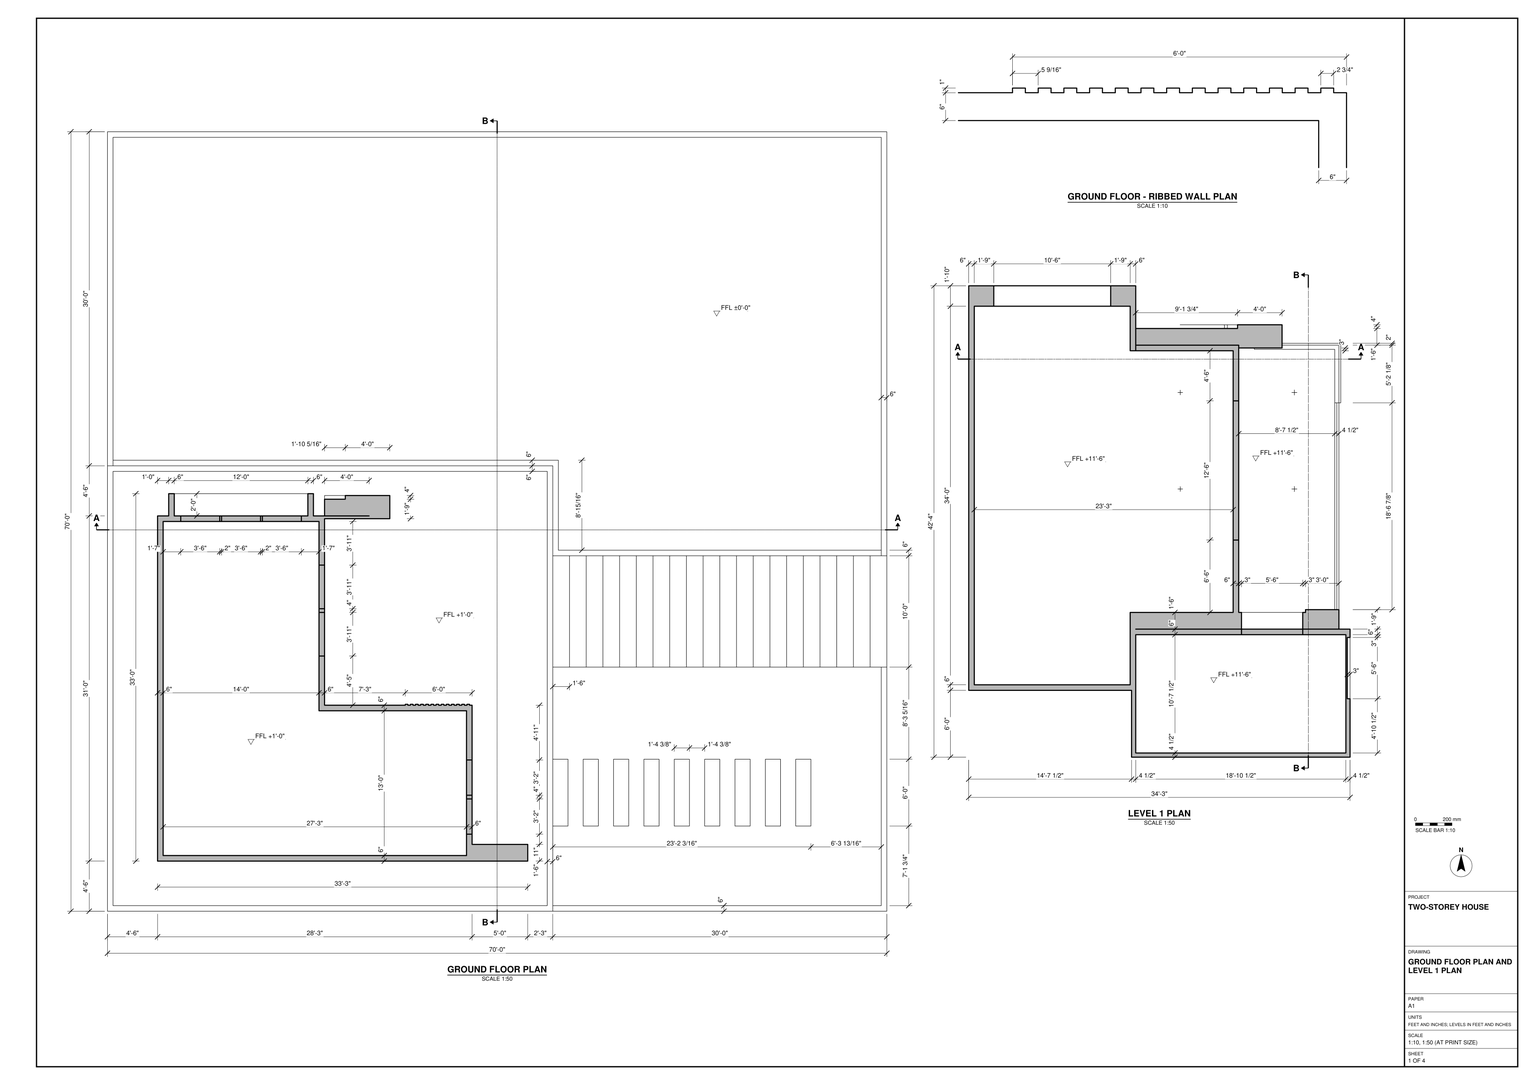
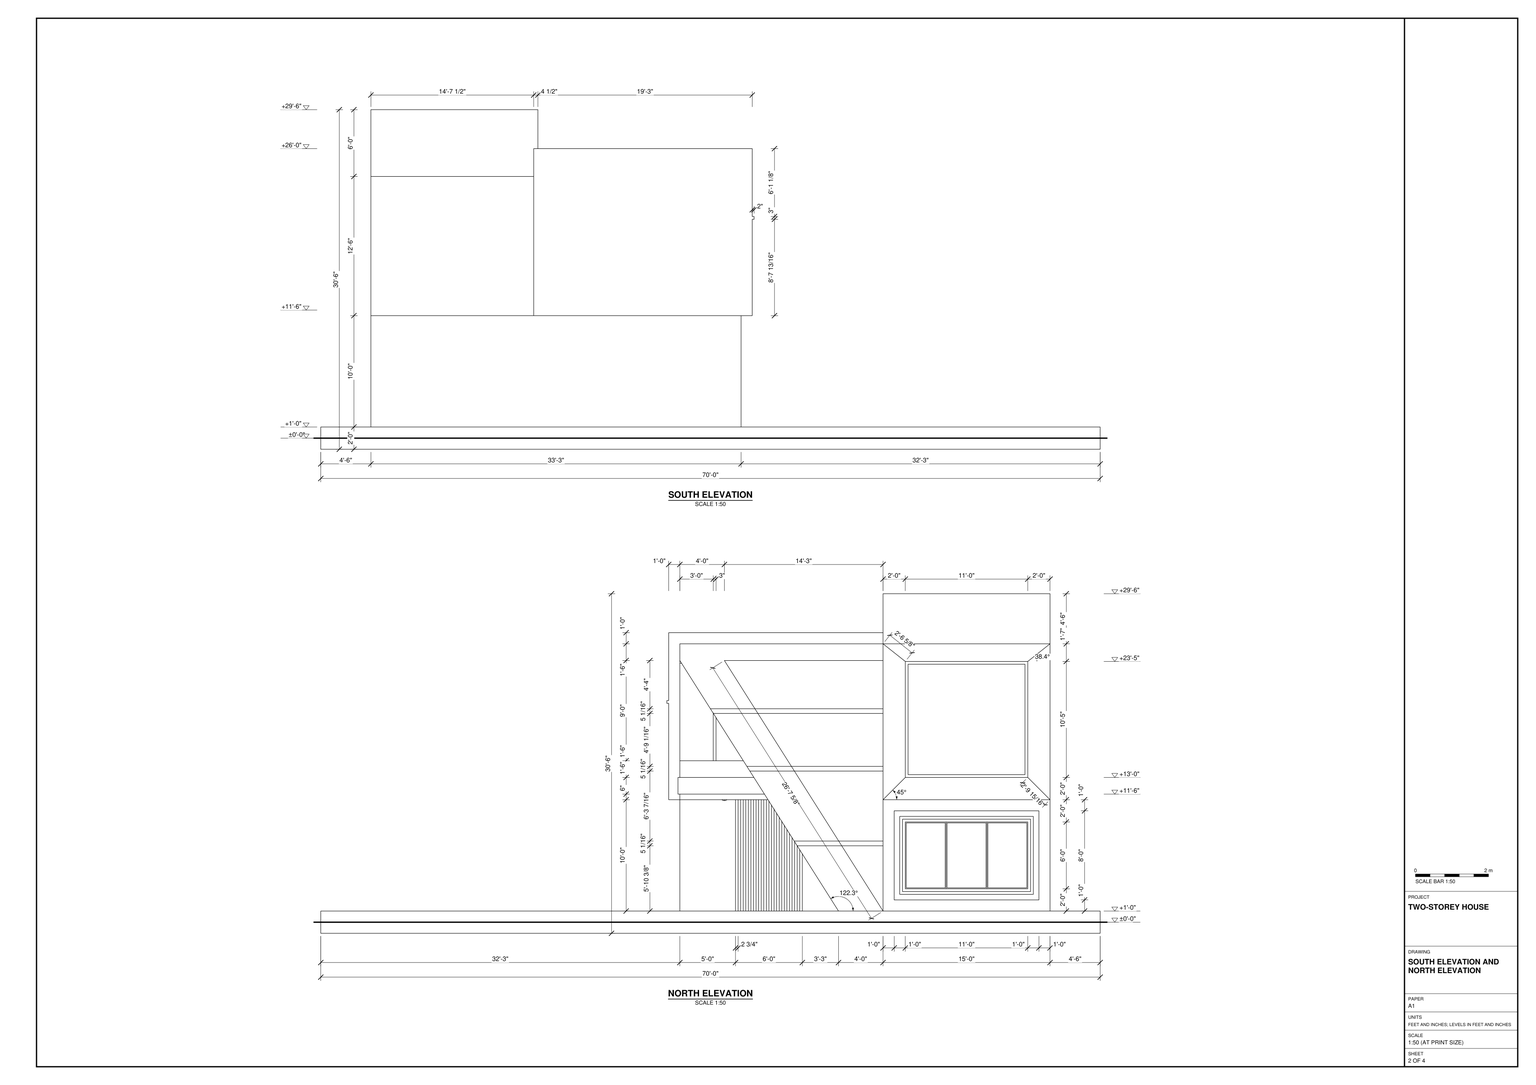
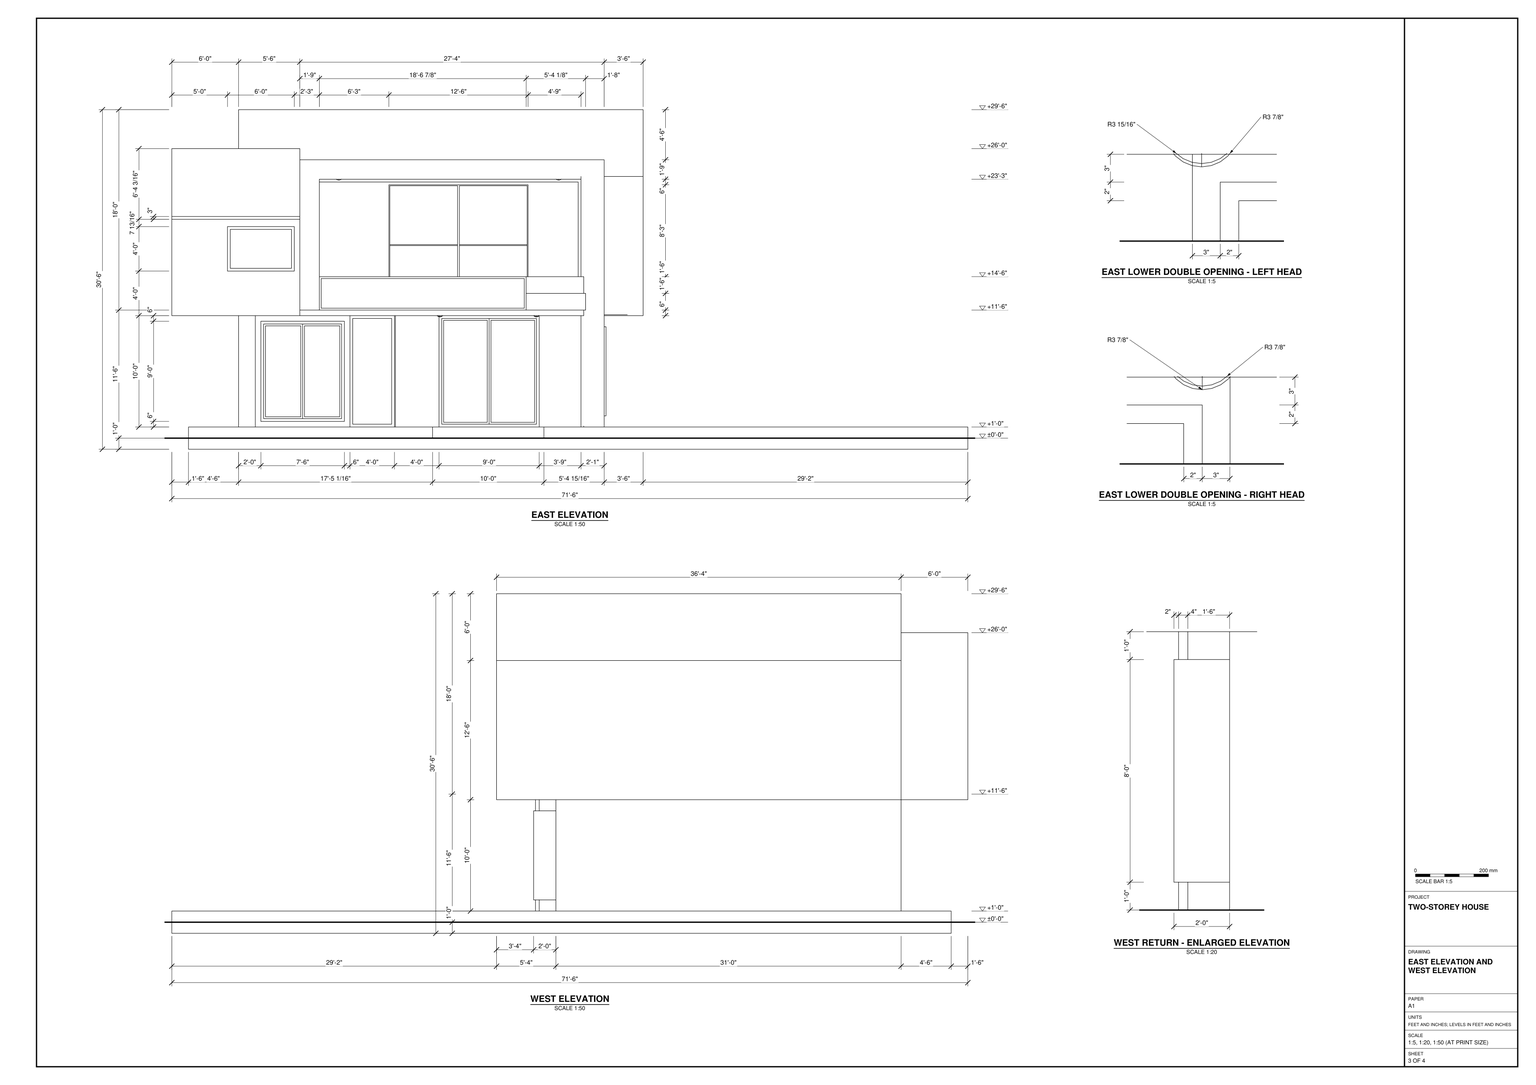
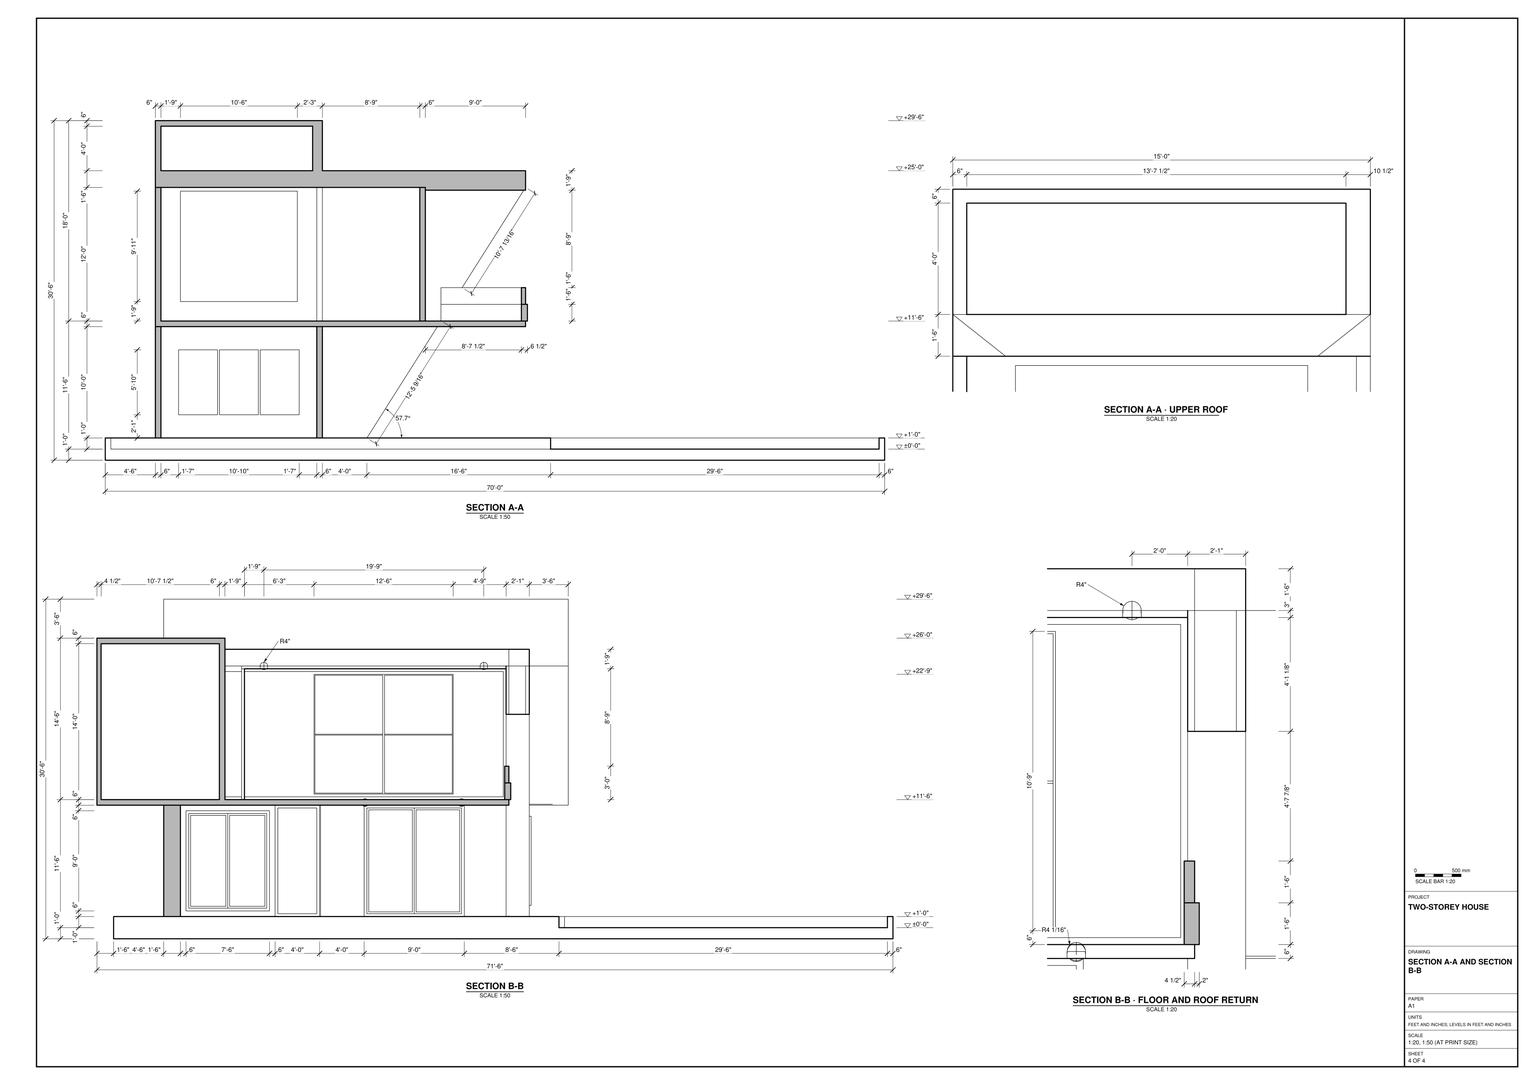
Build the house and its site in SketchUp from task_files/diagram_01.pdf. Work in feet and inches. The complete model, including the base, measures 70'-0" along X, 71'-6" along Y and 30'-6" along Z. Use ±0'-0" as the ground datum, with the raised ground-floor surface at +1'-0" and Level 1 at +11'-6".

Lay out the site edge, raised terrace and two distinct runs of rectangular paving shown in the ground-floor plan. Set the L-shaped lower storey near the southwest corner of the site. Trace the wall thicknesses as drawn, including the ribbed wall at the recess. Use the Level 1 plan for the upper slab and projecting volumes rather than extruding the lower footprint. Form the flat roof sections at their respective heights.

Use the elevations to place the openings and give their frames, reveals and projecting surrounds depth. On the north face, model the diagonal member beside the stacked framed bays. On the east face, distinguish the paired lower openings from the recessed upper opening behind the low balcony wall. Keep the south and west wall faces largely uninterrupted as drawn.

Keep walls, slabs and roof elements in separate groups or components. Keep each furniture or joinery piece shown separate, and use components for repeated parts. Any decor or loose items shown may use suitable library components. Save one SketchUp model as output_files/two_storey_house_with_stepped_roofs_and_raised_terrace.skp.

# SketchUp Ruby script. Lengths in inches.
U = 1.inch
M = Sketchup.active_model
def pt(a) = Geom::Point3d.new(a.map { |v| v * U })
def face(e, loops, mat)
  f = e.add_face(loops[0].map { |a| pt(a) })
  loops[1..].each { |l| e.add_face(l.map { |a| pt(a) }).erase! }
  f.material = f.back_material = mat if mat
  f
end
# faces: each face lists its corners as indices into pts; further lists are holes
def faces(e, pts, list, mat = nil) = list.each { |f| face(e, (f[0].is_a?(Array) ? f : [f]).map { |l| l.map { |i| pts[i] } }, mat) }
# xy, xz, yz: faces in a plane at the given z, y or x. An outline is a flat list of corners, or four numbers for a rectangle; further outlines are holes
def ring(l) = l.size == 4 ? [[l[0], l[1]], [l[2], l[1]], [l[2], l[3]], [l[0], l[3]]] : l.each_slice(2).to_a
def flat(e, list, mat, &to3) = list.each { |f| face(e, (f[0].is_a?(Array) ? f : [f]).map { |l| ring(l).map { |u, v| to3.(u, v) } }, mat) }
def xy(e, z, list, mat = nil) = flat(e, list, mat) { |x, y| [x, y, z] }
def xz(e, y, list, mat = nil) = flat(e, list, mat) { |x, z| [x, y, z] }
def yz(e, x, list, mat = nil) = flat(e, list, mat) { |y, z| [x, y, z] }
def lines(e, pts, list) = list.each { |a, b| e.add_line(pt(pts[a]), pt(pts[b])) }
# prism: a flat outline (further loops are holes) pulled along v
def prism(e, loops, v, mat = nil)
  f = face(e, loops, mat); d = Geom::Vector3d.new(v.map { |x| x * U })
  f.pushpull(f.normal.samedirection?(d) ? d.length : -d.length)
end
def box(e, o, s, mat = nil) = prism(e, [[o, [o[0] + s[0], o[1], o[2]], [o[0] + s[0], o[1] + s[1], o[2]], [o[0], o[1] + s[1], o[2]]]], [0, 0, s[2]], mat)
def at(x, y, z, deg = 0) = Geom::Transformation.translation(pt([x, y, z])) * Geom::Transformation.rotation(ORIGIN, Z_AXIS, deg.degrees)
def axes(o, x, y, z) = Geom::Transformation.new([*x, 0, *y, 0, *z, 0, *pt(o).to_a, 1])
def part(name) = M.definitions.add(name)
# library, detail: a bought-in or finely detailed component or shape, given as its bounding box
def library(name, o, s) = part(name).tap { |d| box(d.entities, o, s) }
def detail(e, o, s) = box(e.add_group.entities, o, s)
def put(e, d, t, mat = nil) = e.add_instance(d, t).tap { |i| i.material = mat if mat }
def group(e, t, mat = nil) = e.add_group.tap { |g| g.transformation = t; g.material = mat if mat }.entities
root = M.entities
M.materials.add("C01_Vanilla_Cream").color = [255, 246, 235]
M.materials.add("D01_Frost_White").color = [255, 251, 241]
M.materials.add("Glass_Basic_01").color = [214, 197, 60]
M.materials["Glass_Basic_01"].alpha = 0.25
M.materials.add("M00_Soft_Cloud").color = [255, 255, 255]
M.materials.add("Metal_10_1K").color = [196, 175, 123]
M.materials.add("Plaster_03_1K").color = [121, 105, 83]
M.materials.add("Plywood_01_1K").color = [125, 96, 64]
M.materials.add("Roofing_02_1K").color = [244, 255, 169]
M.materials.add("Wood_Veneer_15_1K").color = [142, 87, 40]
M.materials.add("Wood_Veneer_15_1K1").color = [103, 69, 45]
c1 = library("Sphere Light",[-4,-4,-4],[8,8,8])
c2 = library("Sphere Light\#1",[-4,-4,-4],[8,8,8])
c3 = library("Sphere Light\#2",[-4,-4,-4],[8,8,8])
c4 = library("Sphere Light\#3",[-4,-4,-4],[8,8,8])
c5 = library("Sphere Light\#4",[-4,-4,-4],[8,8,8])
c6 = library("Sphere Light\#5",[-4,-4,-4],[8,8,8])
c7 = library("Sphere Light\#6",[-3.97,-3.97,-3.97],[7.94,7.94,7.94])
c8 = library("Sphere Light\#7",[-4,-4,-4],[8,8,8])
xz(root,438,[[79,49,121,119],[123,49,165,119],[167,49,209,119]],"Glass_Basic_01")
xz(root,444,[[79,49,121,119],[123,49,165,119],[167,49,209,119]],"Glass_Basic_01")
xz(root,486,[[81,171,207,290]],"Glass_Basic_01")
xz(root,508,[[81,171,207,290]],"Glass_Basic_01")
g1 = group(root,at(0,18,0),"C01_Vanilla_Cream")
xy(g1,0,[[0,0,840,840]])
xy(g1,12,[[480,91.77,496.36,163.77],[512.73,91.77,529.09,163.77],[545.45,91.77,561.82,163.77],[578.18,91.77,594.55,163.77],[610.91,91.77,627.27,163.77],
  [643.64,91.77,660,163.77],[676.36,91.77,692.73,163.77],[709.09,91.77,725.45,163.77],[741.82,91.77,758.18,163.77]],"D01_Frost_White")
xy(g1,12,[[480,263.05,498,383.05],[516,263.05,534,383.05],[552,263.05,570,383.05],[588,263.05,606,383.05],[624,263.05,642,383.05],
  [660,263.05,678,383.05],[696,263.05,714,383.05],[732,263.05,750,383.05],[768,263.05,786,383.05],[804,263.05,822,383.05]],"M00_Soft_Cloud")
xy(g1,12,[[[480,6,834,6,834,263.05,480,263.05,480,163.77,496.36,163.77,496.36,91.77,480,91.77],[512.73,91.77,529.09,163.77],[578.18,91.77,594.55,163.77],[610.91,91.77,627.27,163.77],[643.64,91.77,660,163.77],[676.36,91.77,692.73,163.77],[741.82,91.77,758.18,163.77],[709.09,91.77,725.45,163.77],[545.45,91.77,561.82,163.77]],[498,263.05,516,383.05],[534,263.05,552,383.05],[570,263.05,588,383.05],[606,263.05,624,383.05],
  [642,263.05,660,383.05],[678,263.05,696,383.05],[714,263.05,732,383.05],[750,263.05,768,383.05],[786,263.05,804,383.05],
  [822,263.05,840,383.05],[480,383.05,834,383.05,834,389.05,486,389.05,486,486,6,486,6,480,480,480],[486,389.05,834,389.05,834,834,6,834,6,486,486,486]],"Roofing_02_1K")
xy(g1,24,[[480,0,840,0,840,263.05,834,263.05,834,6,480,6],[834,383.05,840,383.05,840,840,0,840,0,480,6,480,6,834,834,834]],"Plaster_03_1K")
xz(g1,0,[[0,0,840,24]],"Plaster_03_1K")
xz(g1,6,[[480,12,834,24]],"Plaster_03_1K")
xz(g1,263.05,[[834,12,840,24]],"Plaster_03_1K")
xz(g1,383.05,[[834,12,840,24]],"Plaster_03_1K")
xz(g1,480,[[6,12,480,24]])
xz(g1,834,[[6,12,834,24]],"Plaster_03_1K")
xz(g1,840,[[0,0,840,24]],"Plaster_03_1K")
yz(g1,0,[[0,0,840,24]],"Plaster_03_1K")
yz(g1,6,[[486,12,834,24]],"Plaster_03_1K")
yz(g1,6,[[480,12,486,24]],"Roofing_02_1K")
yz(g1,480,[[6,12,480,24]])
yz(g1,834,[[6,12,263.05,24],[389.05,12,834,24]],"Plaster_03_1K")
yz(g1,834,[[383.05,12,389.05,24]],"Roofing_02_1K")
yz(g1,840,[[0,0,840,0,840,24,383.05,24,383.05,12,263.05,12,263.05,24,0,24]],"Plaster_03_1K")
g2 = group(g1,at(0,0,24))
box(g2,[60,60,288],[163.5,408,48])
xy(g2,0,[[[0,0,480,480],[6,6,474,474]],[[6,6,474,474],[54,54,54,426,234,426,234,448,282,448,282,423,234,423,234,222,321,222,321,223,323.77,223,323.77,222,326.54,222,326.54,223,329.31,223,329.31,222,332.08,222,332.08,223,334.85,223,334.85,222,337.62,222,337.62,223,340.38,223,340.38,222,343.15,222,343.15,223,345.92,223,345.92,222,348.69,222,348.69,223,351.46,223,351.46,222,354.23,222,354.23,223,357,223,357,222,359.77,222,359.77,223,362.54,223,362.54,222,365.31,222,365.31,223,368.08,223,368.08,222,370.85,222,370.85,223,373.62,223,373.62,222,376.38,222,376.38,223,379.15,223,379.15,222,381.92,222,381.92,223,384.69,223,384.69,222,387.46,222,387.46,223,390.23,223,390.23,222,393,222,393,72,453,72,453,54]],[54,54,453,54,453,72,393,72,393,222,390.23,222,390.23,223,387.46,223,387.46,222,384.69,222,384.69,223,381.92,223,381.92,222,379.15,222,379.15,223,376.38,223,376.38,222,373.62,222,373.62,223,370.85,223,370.85,222,368.08,222,368.08,223,365.31,223,365.31,222,362.54,222,362.54,223,359.77,223,359.77,222,357,222,357,223,354.23,223,354.23,222,351.46,222,351.46,223,348.69,223,348.69,222,345.92,222,345.92,223,343.15,223,343.15,222,340.38,222,340.38,223,337.62,223,337.62,222,334.85,222,334.85,223,332.08,223,332.08,222,329.31,222,329.31,223,326.54,223,326.54,222,323.77,222,323.77,223,321,223,321,222,234,222,234,420,228,420,228,216,387,216,387,60,60,60,60,420,234,420,234,423,282,423,282,426,54,426],[60,60,387,60,387,216,228,216,228,420,60,420],[234,426,282,448]])
xy(g2,5,[[228,275,234,322],[228,326,234,373]])
xy(g2,11,[[387,83,393,121],[387,125,393,163]])
xy(g2,12,[[66,426,222,450]],"Wood_Veneer_15_1K")
xy(g2,18,[[72,426,216,450]],"Wood_Veneer_15_1K")
xy(g2,25,[[79,420,121,426],[123,420,165,426],[167,420,209,426]])
xy(g2,95,[[79,420,121,426],[123,420,165,426],[167,420,209,426]])
xy(g2,102,[[72,426,216,450]],"Wood_Veneer_15_1K")
xy(g2,108,[[66,426,222,450]],"Wood_Veneer_15_1K")
xy(g2,109,[[387,83,393,121],[387,125,393,163]])
xy(g2,115,[[228,275,234,322],[228,326,234,373]])
xy(g2,120,[[229.5,-18,465,54],[54,54,60,420],[60,54,387,60],[387,54,453,54,453,72,393,72,393,222,390.23,222,390.23,223,387.46,223,387.46,222,387,222],[453,54,465,72],
  [60,60,60,420,228,420,228,216,387,216,387,60],[[393,72,393,222,390.23,222,390.23,223,387.46,223,387.46,222,384.69,222,384.69,223,381.92,223,381.92,222,379.15,222,379.15,223,376.38,223,376.38,222,373.62,222,373.62,223,370.85,223,370.85,222,368.08,222,368.08,223,365.31,223,365.31,222,362.54,222,362.54,223,359.77,223,359.77,222,357,222,357,223,354.23,223,354.23,222,351.46,222,351.46,223,348.69,223,348.69,222,345.92,222,345.92,223,343.15,223,343.15,222,340.38,222,340.38,223,337.62,223,337.62,222,334.85,222,334.85,223,332.08,223,332.08,222,329.31,222,329.31,223,326.54,223,326.54,222,323.77,222,323.77,223,321,223,321,222,234,222,234,423,358,423,358,426,453,426,453,120,465,120,465,72],[281.81,267,282.85,267.09,283.83,267.44,284.69,268.04,285.36,268.84,285.81,269.78,286,270.81,285.98,271,401,271,401.14,269.96,401.54,269,402.17,268.17,403,267.54,403.96,267.14,405,267,406.04,267.14,407,267.54,407.83,268.17,408.46,269,408.86,269.96,409,271,408.86,272.04,408.46,273,407.83,273.83,407,274.46,406.04,274.86,405,275,405,371,406.04,371.14,407,371.54,407.83,372.17,408.46,373,408.86,373.96,409,375,408.86,376.04,408.46,377,407.83,377.83,407,378.46,406.04,378.86,405,379,403.96,378.86,403,378.46,402.17,377.83,401.54,377,401.14,376.04,401,375,286,375,285.86,376.04,285.46,377,284.83,377.83,284,378.46,283.04,378.86,282,379,280.96,378.86,280,378.46,279.17,377.83,278.54,377,278.14,376.04,278,375,278.14,373.96,278.54,373,279.17,372.17,280,371.54,280.96,371.14,282,371,282,274.98,281.15,274.91,280.17,274.56,279.31,273.96,278.64,273.16,278.19,272.22,278,271.19,278.09,270.15,278.44,269.17,279.04,268.31,279.84,267.64,280.78,267.19]],[228,216,387,216,387,222,384.69,222,384.69,223,381.92,223,381.92,222,379.15,222,379.15,223,376.38,223,376.38,222,373.62,222,373.62,223,370.85,223,370.85,222,368.08,222,368.08,223,365.31,223,365.31,222,362.54,222,362.54,223,359.77,223,359.77,222,357,222,357,223,354.23,223,354.23,222,351.46,222,351.46,223,348.69,223,348.69,222,345.92,222,345.92,223,343.15,223,343.15,222,340.38,222,340.38,223,337.62,223,337.62,222,334.85,222,334.85,223,332.08,223,332.08,222,329.31,222,329.31,223,326.54,223,326.54,222,323.77,222,323.77,223,321,223,321,222,234,222,234,423,282,423,282,426,228,426],[285.98,271,285.91,271.85,285.56,272.83,284.96,273.69,284.16,274.36,283.22,274.81,282.19,275,282,274.98,282,371,283.04,371.14,284,371.54,284.83,372.17,285.46,373,285.86,373.96,286,375,401,375,401.14,373.96,401.54,373,402.17,372.17,403,371.54,403.96,371.14,405,371,405,275,403.96,274.86,403,274.46,402.17,273.83,401.54,273,401.14,272.04,401,271],[54,420,228,426],
  [282,423,353.25,426],[353.25,423,358,426],[54,426,234,490]])
xy(g2,122.65,[[281.81,267,280.78,267.19,279.84,267.64,279.04,268.31,278.44,269.17,278.09,270.15,278,271.19,278.19,272.22,278.64,273.16,279.31,273.96,280.17,274.56,281.15,274.91,282,274.98,282,271,285.98,271,286,270.81,285.81,269.78,285.36,268.84,284.69,268.04,283.83,267.44,282.85,267.09],[282,271,282,274.98,282.19,275,283.22,274.81,284.16,274.36,284.96,273.69,285.56,272.83,285.91,271.85,285.98,271],[282,371,280.96,371.14,280,371.54,279.17,372.17,278.54,373,278.14,373.96,278,375,278.14,376.04,278.54,377,279.17,377.83,280,378.46,280.96,378.86,282,379,283.04,378.86,284,378.46,284.83,377.83,285.46,377,285.86,376.04,286,375,282,375],[282,371,282,375,286,375,285.86,373.96,285.46,373,284.83,372.17,284,371.54,283.04,371.14]])
xy(g2,123,[[405,267,403.96,267.14,403,267.54,402.17,268.17,401.54,269,401.14,269.96,401,271,405,271,405,275,406.04,274.86,407,274.46,407.83,273.83,408.46,273,408.86,272.04,409,271,408.86,269.96,408.46,269,407.83,268.17,407,267.54,406.04,267.14],[401,271,401.14,272.04,401.54,273,402.17,273.83,403,274.46,403.96,274.86,405,275,405,271],[405,371,403.96,371.14,403,371.54,402.17,372.17,401.54,373,401.14,373.96,401,375,405,375],[405,371,405,375,401,375,401.14,376.04,401.54,377,402.17,377.83,403,378.46,403.96,378.86,405,379,406.04,378.86,407,378.46,407.83,377.83,408.46,377,408.86,376.04,409,375,408.86,373.96,408.46,373,407.83,372.17,407,371.54,406.04,371.14]])
xy(g2,126,[[234,-13.5,460.5,114],[60,60,228,60,228,138,339,138,339,420,228,420,228,468,60,468],[234,120,453,120,453,141,417,141,417,138,345,138,345,426,234,426,234,420,339,420,339,138,234,138],[345,138,417,138,417,141,448.5,141,448.5,421.5,361.8,421.5,361.8,423,345,423],[448.5,141,450.75,363.9],
  [450.75,141,453,363.9],[448.5,363.9,448.5,421.5,361.8,421.5,361.8,426,453,426,453,363.9],[345,423,356.8125,426],[356.8125,423,361.8,426]])
xy(g2,126,[[453,363.9,455,426],[361.8,426,455,428]],"C01_Vanilla_Cream")
xy(g2,128,[[448.5,143,450.75,361.9]])
xy(g2,129,[[348,114,414,120],[348,120,414,138]])
xy(g2,132,[[339,216,345,366]])
xy(g2,144,[[448.5,363.9,448.5,421.5,361.8,421.5,361.8,426,453,426,453,363.9]])
xy(g2,144,[[453,363.9,455,363.9,455,428,373.2,428,373.2,426,453,426]],"C01_Vanilla_Cream")
xy(g2,147,[[81,468,207,490]],"C01_Vanilla_Cream")
xy(g2,160,[[448.5,143,450.75,361.9]])
xy(g2,162,[[448.5,141,450.75,363.9],[448.5,363.9,453,363.9,453,426,384.6,426,384.6,423,361.8,423,361.8,421.5,448.5,421.5],[361.8,423,384.6,426]])
xy(g2,171,[[462.01,45,465,111]])
xy(g2,213,[[462.01,45,465,111]])
xy(g2,223.83,[[465,-18,467,120]])
xy(g2,226.85,[[465,-18,467,120]])
xy(g2,261,[[339,216,345,366]])
xy(g2,264,[[348,114,414,120],[348,120,414,138]])
xy(g2,266,[[81,468,207,490]])
xy(g2,267,[[[345,138,345,423,453,423,453,141,417,141,417,138],[429,158,430.04,158.14,431,158.54,431.83,159.17,432.46,160,432.86,160.96,433,162,432.86,163.04,432.46,164,431.83,164.83,431,165.46,430.04,165.86,429,166,427.96,165.86,427,165.46,426.17,164.83,425.54,164,425.14,163.04,425,162,425.14,160.96,425.54,160,426.17,159.17,427,158.54,427.96,158.14],[369,158,370.04,158.14,371,158.54,371.83,159.17,372.46,160,372.86,160.96,373,162,372.86,163.04,372.46,164,371.83,164.83,371,165.46,370.04,165.86,369,166,367.96,165.86,367,165.46,366.17,164.83,365.54,164,365.14,163.04,365,162,365.14,160.96,365.54,160,366.17,159.17,367,158.54,367.96,158.14],[429,395,430.04,395.14,431,395.54,431.83,396.17,432.46,397,432.86,397.96,433,399,432.86,400.04,432.46,401,431.83,401.83,431,402.46,430.04,402.86,429,403,427.96,402.86,427,402.46,426.17,401.83,425.54,401,425.14,400.04,425,399,425.14,397.96,425.54,397,426.17,396.17,427,395.54,427.96,395.14],[369,395,370.04,395.14,371,395.54,371.83,396.17,372.46,397,372.86,397.96,373,399,372.86,400.04,372.46,401,371.83,401.83,371,402.46,370.04,402.86,369,403,367.96,402.86,367,402.46,366.17,401.83,365.54,401,365.14,400.04,365,399,365.14,397.96,365.54,397,366.17,396.17,367,395.54,367.96,395.14]]],"D01_Frost_White")
xy(g2,270,[[54,54,228,60],[54,60,60,120],[60,60,60,468,228,468,228,420,339,420,339,138,228,138,228,60],[54,120,60,138],[234,120,339,138],
  [339,120,339,420,234,420,234,426,345,426,345,120],[54,138,60,426],[54,426,60,468]])
xy(g2,270,[[369,158,367.96,158.14,367,158.54,366.17,159.17,365.54,160,365.14,160.96,365,162,365.14,163.04,365.54,164,366.17,164.83,367,165.46,367.96,165.86,369,166,369,162,373,162,372.86,160.96,372.46,160,371.83,159.17,371,158.54,370.04,158.14],[429,158,427.96,158.14,427,158.54,426.17,159.17,425.54,160,425.14,160.96,425,162,429,162,429,166,430.04,165.86,431,165.46,431.83,164.83,432.46,164,432.86,163.04,433,162,432.86,160.96,432.46,160,431.83,159.17,431,158.54,430.04,158.14],[369,162,369,166,370.04,165.86,371,165.46,371.83,164.83,372.46,164,372.86,163.04,373,162],[425,162,425.14,163.04,425.54,164,426.17,164.83,427,165.46,427.96,165.86,429,166,429,162],[369,395,367.96,395.14,367,395.54,366.17,396.17,365.54,397,365.14,397.96,365,399,365.14,400.04,365.54,401,366.17,401.83,367,402.46,367.96,402.86,369,403],
  [369,395,369,399,373,399,372.86,397.96,372.46,397,371.83,396.17,371,395.54,370.04,395.14],[429,395,427.96,395.14,427,395.54,426.17,396.17,425.54,397,425.14,397.96,425,399,429,399],[429,395,429,403,430.04,402.86,431,402.46,431.83,401.83,432.46,401,432.86,400.04,433,399,432.86,397.96,432.46,397,431.83,396.17,431,395.54,430.04,395.14],[369,399,369,403,370.04,402.86,371,402.46,371.83,401.83,372.46,401,372.86,400.04,373,399],[425,399,425.14,400.04,425.54,401,426.17,401.83,427,402.46,427.96,402.86,429,403,429,399],
  [234,444,405,448]],"D01_Frost_White")
xy(g2,288,[[234,120,453,448]],"D01_Frost_White")
xy(g2,294,[[234,-13.5,460.5,114]])
xy(g2,300,[[229.5,-18,465,-18,465,120,234,120,234,54,229.5,54]],"C01_Vanilla_Cream")
xy(g2,342,[[54,54,234,490]],"C01_Vanilla_Cream")
xz(g2,-18,[[229.5,120,465,120,465,223.83,467,223.83,467,226.85,465,226.85,465,300,229.5,300]],"C01_Vanilla_Cream")
xz(g2,-13.5,[[234,126,238.5,294],[238.5,126,460.5,294]])
xz(g2,45,[[462.01,171,465,213]])
xz(g2,54,[[54,0,453,120],[54,120,229.5,270],[54,270,229.5,270,229.5,300,234,300,234,342,54,342]],"C01_Vanilla_Cream")
xz(g2,60,[[60,0,387,120],[60,126,228,270]])
xz(g2,72,[[393,0,453,120]],"C01_Vanilla_Cream")
xz(g2,83,[[387,11,393,109]])
xz(g2,111,[[462.01,171,465,213]])
xz(g2,114,[[[234,126,460.5,294],[348,129,414,264]]])
xz(g2,114,[[348,129,414,264]],"Glass_Basic_01")
xz(g2,120,[[[234,126,453,126,453,288,345,288,345,270,234,270],[348,129,414,264]],[229.5,288,234,300]])
xz(g2,120,[[453,120,453,288,234,288,234,300,465,300,465,226.85,467,226.85,467,223.83,465,223.83,465,120]],"C01_Vanilla_Cream")
xz(g2,120,[[348,129,414,264]],"Glass_Basic_01")
xz(g2,121,[[387,11,393,109]])
xz(g2,125,[[387,11,393,109]])
xz(g2,138,[[228,126,339,270]])
xz(g2,138,[[[345,126,417,267],[348,129,414,264]]],"Wood_Veneer_15_1K1")
xz(g2,141,[[448.5,126,450.75,162]])
xz(g2,141,[[417,126,417,267,453,267,453,126,450.75,126,450.75,162,448.5,162,448.5,126]],"D01_Frost_White")
xz(g2,143,[[448.5,128,450.75,160]])
xz(g2,163,[[387,11,393,109]])
xz(g2,216,[[228,0,387,120],[339,132,345,261]])
xz(g2,222,[[234,0,321,120],[323.77,0,326.54,120],[329.31,0,332.08,120],[334.85,0,337.62,120],[340.38,0,343.15,120],
  [345.92,0,348.69,120],[351.46,0,354.23,120],[357,0,359.77,120],[362.54,0,365.31,120],[368.08,0,370.85,120],
  [373.62,0,376.38,120],[379.15,0,381.92,120],[384.69,0,387.46,120],[390.23,0,393,120]],"Wood_Veneer_15_1K")
xz(g2,223,[[321,0,323.77,120],[326.54,0,329.31,120],[332.08,0,334.85,120],[337.62,0,340.38,120],[343.15,0,345.92,120],
  [348.69,0,351.46,120],[354.23,0,357,120],[359.77,0,362.54,120],[365.31,0,368.08,120],[370.85,0,373.62,120],
  [376.38,0,379.15,120],[381.92,0,384.69,120],[387.46,0,390.23,120]],"Wood_Veneer_15_1K")
xz(g2,275,[[228,5,234,115]])
xz(g2,322,[[228,5,234,115]])
xz(g2,326,[[228,5,234,115]])
xz(g2,361.9,[[448.5,128,450.75,144],[448.5,144,450.75,160]])
xz(g2,363.9,[[448.5,126,450.75,144],[450.75,126,455,144],[448.5,144,450.75,162],[450.75,144,453,162]])
xz(g2,366,[[339,132,345,261]])
xz(g2,373,[[228,5,234,115]])
xz(g2,420,[[[60,0,228,120],[79,25,121,95],[167,25,209,95],[123,25,165,95]],[228,126,234,270],[234,126,339,270]])
xz(g2,421.5,[[361.8,126,448.5,144],[361.8,144,448.5,162]])
xz(g2,423,[[361.8,126,384.6,162,361.8,162],[345,267,442.3125,270],[442.3125,267,451.1,267,453,270,442.3125,270],[451.1,267,453,270,453,267]])
xz(g2,423,[[234,0,282,0,358,120,234,120],[345,126,361.8,126,361.8,162,384.6,162,451.1,267,345,267]],"D01_Frost_White")
xz(g2,426,[[234,0,282,120],[[78,24,122,96],[79,25,121,95]],[[122,24,166,96],[123,25,165,95]],[[166,24,210,96],[167,25,209,95]],[234,120,234,126,356.8125,126,353.25,120],
  [353.25,120,356.8125,126,361.8,126,358,120],[358,120,361.8,126,453,126,453,120],[234,126,345,270],[361.8,126,361.8,144,373.2,144],[361.8,144,361.8,162,384.6,162,373.2,144]])
xz(g2,426,[[[54,0,234,120],[66,12,222,108]],[373.2,144,384.6,162,453,162,453,144]],"C01_Vanilla_Cream")
xz(g2,426,[[[72,18,216,102],[75,21,213,99]],[[75,21,213,99],[78,24,210,96]]],"Wood_Veneer_15_1K")
xz(g2,428,[[361.8,126,373.2,144,455,144,455,126]],"C01_Vanilla_Cream")
xz(g2,444,[[234,0,234,70.35,278.56,70.35],[234,75.42,234,150.84,329.53,150.84,281.77,75.42],[234,155.91,234,212.95,368.87,212.95,332.74,155.91],[234,218.02,234,270,405,270,372.08,218.02]],"D01_Frost_White")
xz(g2,444,[[234,70.35,234,75.42,281.77,75.42,278.56,70.35],[234,150.84,234,155.91,332.74,155.91,329.53,150.84],[234,212.95,234,218.02,372.08,218.02,368.87,212.95]],"Metal_10_1K")
xz(g2,448,[[234,0,278.56,70.35,326.56,70.35,282,0],[281.77,75.42,329.53,150.84,377.53,150.84,329.77,75.42],[332.74,155.91,368.87,212.95,416.87,212.95,380.74,155.91],[372.08,218.02,405,270,234,270,234,288,453,288,453,270,420.08,218.02]],"D01_Frost_White")
xz(g2,448,[[278.56,70.35,281.77,75.42,329.77,75.42,326.56,70.35],[329.53,150.84,332.74,155.91,380.74,155.91,377.53,150.84],[368.87,212.95,372.08,218.02,420.08,218.02,416.87,212.95]],"Metal_10_1K")
xz(g2,450,[[[66,12,222,108],[72,18,216,102]]],"Wood_Veneer_15_1K")
xz(g2,468,[[[60,126,228,270],[81,147,207,266]]])
xz(g2,490,[[54,120,54,288,78,269,78,144],[54,120,78,144,210,144,234,120],[234,120,210,144,210,269,234,288],[78,269,54,288,234,288,210,269],[54,288,234,342]],"C01_Vanilla_Cream")
xz(g2,490,[[[78,144,210,269],[81,147,207,266]]],"Metal_10_1K")
yz(g2,54,[[54,0,426,120],[54,120,490,270],[54,270,490,342]],"C01_Vanilla_Cream")
yz(g2,60,[[60,0,420,120],[60,126,468,270]])
yz(g2,66,[[426,12,450,108]],"Wood_Veneer_15_1K")
yz(g2,72,[[426,18,450,102]],"Wood_Veneer_15_1K")
yz(g2,79,[[420,25,426,95]])
yz(g2,81,[[468,147,490,266]],"C01_Vanilla_Cream")
yz(g2,121,[[420,25,426,95]])
yz(g2,123,[[420,25,426,95]])
yz(g2,165,[[420,25,426,95]])
yz(g2,167,[[420,25,426,95]])
yz(g2,207,[[468,147,490,266]],"C01_Vanilla_Cream")
yz(g2,209,[[420,25,426,95]])
yz(g2,216,[[426,18,450,102]],"Wood_Veneer_15_1K")
yz(g2,222,[[426,12,450,108]],"Wood_Veneer_15_1K")
yz(g2,228,[[[216,0,420,120],[275,5,322,115],[326,5,373,115]],[60,126,138,270],[420,126,426,270],[426,126,468,270]])
yz(g2,228,[[275,5,322,115],[326,5,373,115]],"Glass_Basic_01")
yz(g2,229.5,[[-18,120,54,300]],"C01_Vanilla_Cream")
yz(g2,234,[[426,0,444,120],[426,120,444,270],[-13.5,126,114,294],[420,126,426,270]])
yz(g2,234,[[448,270,490,270,490,342,54,342,54,300,120,300,120,288,448,288]],"C01_Vanilla_Cream")
yz(g2,234,[[275,5,322,115],[326,5,373,115]],"Glass_Basic_01")
yz(g2,234,[[222,0,270,120],[[270,0,378,120],[273,3,375,117]],[378,0,423,120],[444,120,490,270]],"Wood_Veneer_15_1K")
yz(g2,234,[[[273,3,324,117],[275,5,322,115]],[[324,3,375,117],[326,5,373,115]]],"Wood_Veneer_15_1K1")
yz(g2,321,[[222,0,223,120]],"Wood_Veneer_15_1K")
yz(g2,323.77,[[222,0,223,120]],"Wood_Veneer_15_1K")
yz(g2,326.54,[[222,0,223,120]],"Wood_Veneer_15_1K")
yz(g2,329.31,[[222,0,223,120]],"Wood_Veneer_15_1K")
yz(g2,332.08,[[222,0,223,120]],"Wood_Veneer_15_1K")
yz(g2,334.85,[[222,0,223,120]],"Wood_Veneer_15_1K")
yz(g2,337.62,[[222,0,223,120]],"Wood_Veneer_15_1K")
yz(g2,339,[[[138,126,420,270],[216,132,366,261]]])
yz(g2,339,[[216,132,366,261]],"Glass_Basic_01")
yz(g2,340.38,[[222,0,223,120]],"Wood_Veneer_15_1K")
yz(g2,343.15,[[222,0,223,120]],"Wood_Veneer_15_1K")
yz(g2,345,[[423,126,426,270],[138,267,423,270]])
yz(g2,345,[[217,133,290,195.5],[292,133,365,195.5],[217,196.5,290,260],[292,196.5,365,260]],"Glass_Basic_01")
yz(g2,345,[[[216,132,366,261],[292,133,365,260],[217,133,290,260]],[217,195.5,290,196.5],[292,195.5,365,196.5]],"Metal_10_1K")
yz(g2,345,[[[138,126,423,267],[141,129,420,264]]],"Plywood_01_1K")
yz(g2,345,[[[141,129,420,264],[216,132,366,261]]],"Wood_Veneer_15_1K")
yz(g2,345.92,[[222,0,223,120]],"Wood_Veneer_15_1K")
yz(g2,348,[[114,129,120,264]])
yz(g2,348,[[120,129,138,264]],"C01_Vanilla_Cream")
yz(g2,348.69,[[222,0,223,120]],"Wood_Veneer_15_1K")
yz(g2,351.46,[[222,0,223,120]],"Wood_Veneer_15_1K")
yz(g2,354.23,[[222,0,223,120]],"Wood_Veneer_15_1K")
yz(g2,357,[[222,0,223,120]],"Wood_Veneer_15_1K")
yz(g2,359.77,[[222,0,223,120]],"Wood_Veneer_15_1K")
yz(g2,361.8,[[421.5,126,423,144],[423,126,426,144],[421.5,144,423,162],[423,144,426,162]])
yz(g2,362.54,[[222,0,223,120]],"Wood_Veneer_15_1K")
yz(g2,365.31,[[222,0,223,120]],"Wood_Veneer_15_1K")
yz(g2,368.08,[[222,0,223,120]],"Wood_Veneer_15_1K")
yz(g2,370.85,[[222,0,223,120]],"Wood_Veneer_15_1K")
yz(g2,373.62,[[222,0,223,120]],"Wood_Veneer_15_1K")
yz(g2,376.38,[[222,0,223,120]],"Wood_Veneer_15_1K")
yz(g2,379.15,[[222,0,223,120]],"Wood_Veneer_15_1K")
yz(g2,381.92,[[222,0,223,120]],"Wood_Veneer_15_1K")
yz(g2,384.69,[[222,0,223,120]],"Wood_Veneer_15_1K")
yz(g2,387,[[[60,0,216,120],[83,11,121,109],[125,11,163,109]]])
yz(g2,387,[[83,11,121,109],[125,11,163,109]],"Glass_Basic_01")
yz(g2,387.46,[[222,0,223,120]],"Wood_Veneer_15_1K")
yz(g2,390.23,[[222,0,223,120]],"Wood_Veneer_15_1K")
yz(g2,393,[[[72,0,174,120],[78,6,168,114]],[177,3,219,117]],"C01_Vanilla_Cream")
yz(g2,393,[[83,11,121,109],[125,11,163,109]],"Glass_Basic_01")
yz(g2,393,[[[78,6,168,114],[81,9,165,111]]],"Wood_Veneer_15_1K")
yz(g2,393,[[[174,0,222,120],[177,3,219,117]],[[81,9,123,111],[83,11,121,109]],[[123,9,165,111],[125,11,163,109]]],"Wood_Veneer_15_1K1")
yz(g2,414,[[114,129,120,264],[120,129,138,264]])
yz(g2,417,[[138,126,141,267]])
yz(g2,448.5,[[[141,126,363.9,162],[143,128,361.9,160]],[363.9,126,421.5,144],[363.9,144,421.5,162]])
yz(g2,448.5,[[143,128,361.9,160]],"Glass_Basic_01")
yz(g2,450.75,[[143,128,361.9,160]],"Glass_Basic_01")
yz(g2,450.75,[[[141,126,363.9,162],[143,128,361.9,160]]],"Metal_10_1K")
yz(g2,453,[[120,120,426,126]])
yz(g2,453,[[54,0,72,120],[363.9,144,426,162]],"C01_Vanilla_Cream")
yz(g2,453,[[120,126,141,126,141,267,423,267,423,270,448,270,448,288,120,288]],"D01_Frost_White")
yz(g2,455,[[363.9,126,428,144]],"C01_Vanilla_Cream")
yz(g2,460.5,[[-13.5,126,114,294]])
yz(g2,462.01,[[45,171,111,213]],"C01_Vanilla_Cream")
yz(g2,465,[[[42,168,114,216],[45,171,111,213]]])
yz(g2,465,[[[-18,120,120,223.83],[42,168,114,216]],[-18,226.85,120,300]],"C01_Vanilla_Cream")
yz(g2,467,[[-18,223.83,120,226.85]])
p = [[451.1,423,267],[384.6,423,162],[384.6,426,162],[373.2,426,144],[373.2,428,144],[361.8,428,126],
  [361.8,426,126],[358,426,120],[358,423,120],[282,423,0],[282,426,0],[282,448,0],
  [326.56,448,70.35],[329.77,448,75.42],[377.53,448,150.84],[380.74,448,155.91],[416.87,448,212.95],[420.08,448,218.02],
  [453,448,270],[453,423,270],[234,444,0],[278.56,444,70.35],[278.56,448,70.35],[234,448,0],
  [281.77,444,75.42],[281.77,448,75.42],[329.53,444,150.84],[329.53,448,150.84],[281.81,267,120],[280.78,267.19,120],
  [280.78,267.19,122.65],[281.81,267,122.65],[282.85,267.09,120],[282.85,267.09,122.65],[405,267,120],[403.96,267.14,120],
  [403.96,267.14,123],[405,267,123],[406.04,267.14,120],[406.04,267.14,123],[283.83,267.44,120],[283.83,267.44,122.65],
  [403,267.54,120],[403,267.54,123],[407,267.54,120],[407,267.54,123],[279.84,267.64,120],[279.84,267.64,122.65],
  [284.69,268.04,120],[284.69,268.04,122.65],[402.17,268.17,120],[402.17,268.17,123],[407.83,268.17,120],[407.83,268.17,123],
  [279.04,268.31,120],[279.04,268.31,122.65],[285.36,268.84,120],[285.36,268.84,122.65],[401.54,269,120],[401.54,269,123],
  [408.46,269,120],[408.46,269,123],[278.44,269.17,120],[278.44,269.17,122.65],[285.81,269.78,120],[285.81,269.78,122.65],
  [401.14,269.96,120],[401.14,269.96,123],[408.86,269.96,120],[408.86,269.96,123],[278.09,270.15,120],[278.09,270.15,122.65],
  [286,270.81,120],[286,270.81,122.65],[401,271,120],[401,271,123],[409,271,120],[409,271,123],
  [278,271.19,120],[278,271.19,122.65],[285.98,271,120],[285.98,271,122.65],[285.91,271.85,120],[285.91,271.85,122.65],
  [401.14,272.04,120],[401.14,272.04,123],[408.86,272.04,120],[408.86,272.04,123],[278.19,272.22,120],[278.19,272.22,122.65],
  [285.56,272.83,120],[285.56,272.83,122.65],[401.54,273,120],[401.54,273,123],[408.46,273,120],[408.46,273,123],
  [278.64,273.16,120],[278.64,273.16,122.65],[284.96,273.69,120],[284.96,273.69,122.65],[402.17,273.83,120],[402.17,273.83,123],
  [407.83,273.83,120],[407.83,273.83,123],[279.31,273.96,120],[279.31,273.96,122.65],[284.16,274.36,120],[284.16,274.36,122.65],
  [403,274.46,120],[403,274.46,123],[407,274.46,120],[407,274.46,123],[280.17,274.56,120],[280.17,274.56,122.65],
  [283.22,274.81,120],[283.22,274.81,122.65],[403.96,274.86,120],[403.96,274.86,123],[406.04,274.86,120],[406.04,274.86,123],
  [281.15,274.91,120],[281.15,274.91,122.65],[282.19,275,120],[282.19,275,122.65],[282,274.98,120],[282,274.98,122.65],
  [405,275,120],[405,275,123],[282,371,120],[280.96,371.14,120],[280.96,371.14,122.65],[282,371,122.65],
  [283.04,371.14,120],[283.04,371.14,122.65],[405,371,120],[403.96,371.14,120],[403.96,371.14,123],[405,371,123],
  [406.04,371.14,120],[406.04,371.14,123],[280,371.54,120],[280,371.54,122.65],[284,371.54,120],[284,371.54,122.65],
  [403,371.54,120],[403,371.54,123],[407,371.54,120],[407,371.54,123],[279.17,372.17,120],[279.17,372.17,122.65],
  [284.83,372.17,120],[284.83,372.17,122.65],[402.17,372.17,120],[402.17,372.17,123],[407.83,372.17,120],[407.83,372.17,123],
  [278.54,373,120],[278.54,373,122.65],[285.46,373,120],[285.46,373,122.65],[401.54,373,120],[401.54,373,123],
  [408.46,373,120],[408.46,373,123],[278.14,373.96,120],[278.14,373.96,122.65],[285.86,373.96,120],[285.86,373.96,122.65],
  [401.14,373.96,120],[401.14,373.96,123],[408.86,373.96,120],[408.86,373.96,123],[278,375,120],[278,375,122.65],
  [286,375,120],[286,375,122.65],[401,375,120],[401,375,123],[409,375,120],[409,375,123],
  [278.14,376.04,120],[278.14,376.04,122.65],[285.86,376.04,120],[285.86,376.04,122.65],[401.14,376.04,120],[401.14,376.04,123],
  [408.86,376.04,120],[408.86,376.04,123],[278.54,377,120],[278.54,377,122.65],[285.46,377,120],[285.46,377,122.65],
  [401.54,377,120],[401.54,377,123],[408.46,377,120],[408.46,377,123],[279.17,377.83,120],[279.17,377.83,122.65],
  [284.83,377.83,120],[284.83,377.83,122.65],[402.17,377.83,120],[402.17,377.83,123],[407.83,377.83,120],[407.83,377.83,123],
  [280,378.46,120],[280,378.46,122.65],[284,378.46,120],[284,378.46,122.65],[403,378.46,120],[403,378.46,123],
  [407,378.46,120],[407,378.46,123],[280.96,378.86,120],[280.96,378.86,122.65],[283.04,378.86,120],[283.04,378.86,122.65],
  [403.96,378.86,120],[403.96,378.86,123],[406.04,378.86,120],[406.04,378.86,123],[282,379,120],[282,379,122.65],
  [405,379,120],[405,379,123],[361.8,423,126],[332.74,444,155.91],[332.74,448,155.91],[368.87,444,212.95],
  [368.87,448,212.95],[372.08,444,218.02],[372.08,448,218.02],[405,444,270],[405,448,270],[369,158,267],
  [367.96,158.14,267],[367.96,158.14,270],[369,158,270],[370.04,158.14,267],[370.04,158.14,270],[429,158,267],
  [427.96,158.14,267],[427.96,158.14,270],[429,158,270],[430.04,158.14,267],[430.04,158.14,270],[367,158.54,267],
  [367,158.54,270],[371,158.54,267],[371,158.54,270],[427,158.54,267],[427,158.54,270],[431,158.54,267],
  [431,158.54,270],[366.17,159.17,267],[366.17,159.17,270],[371.83,159.17,267],[371.83,159.17,270],[426.17,159.17,267],
  [426.17,159.17,270],[431.83,159.17,267],[431.83,159.17,270],[365.54,160,267],[365.54,160,270],[372.46,160,267],
  [372.46,160,270],[425.54,160,267],[425.54,160,270],[432.46,160,267],[432.46,160,270],[365.14,160.96,267],
  [365.14,160.96,270],[372.86,160.96,267],[372.86,160.96,270],[425.14,160.96,267],[425.14,160.96,270],[432.86,160.96,267],
  [432.86,160.96,270],[365,162,267],[365,162,270],[373,162,267],[373,162,270],[425,162,267],
  [425,162,270],[433,162,267],[433,162,270],[365.14,163.04,267],[365.14,163.04,270],[372.86,163.04,267],
  [372.86,163.04,270],[425.14,163.04,267],[425.14,163.04,270],[432.86,163.04,267],[432.86,163.04,270],[365.54,164,267],
  [365.54,164,270],[372.46,164,267],[372.46,164,270],[425.54,164,267],[425.54,164,270],[432.46,164,267],
  [432.46,164,270],[366.17,164.83,267],[366.17,164.83,270],[371.83,164.83,267],[371.83,164.83,270],[426.17,164.83,267],
  [426.17,164.83,270],[431.83,164.83,267],[431.83,164.83,270],[367,165.46,267],[367,165.46,270],[371,165.46,267],
  [371,165.46,270],[427,165.46,267],[427,165.46,270],[431,165.46,267],[431,165.46,270],[367.96,165.86,267],
  [367.96,165.86,270],[370.04,165.86,267],[370.04,165.86,270],[427.96,165.86,267],[427.96,165.86,270],[430.04,165.86,267],
  [430.04,165.86,270],[369,166,267],[369,166,270],[429,166,267],[429,166,270],[369,395,267],
  [367.96,395.14,267],[367.96,395.14,270],[369,395,270],[370.04,395.14,267],[370.04,395.14,270],[429,395,267],
  [427.96,395.14,267],[427.96,395.14,270],[429,395,270],[430.04,395.14,267],[430.04,395.14,270],[367,395.54,267],
  [367,395.54,270],[371,395.54,267],[371,395.54,270],[427,395.54,267],[427,395.54,270],[431,395.54,267],
  [431,395.54,270],[366.17,396.17,267],[366.17,396.17,270],[371.83,396.17,267],[371.83,396.17,270],[426.17,396.17,267],
  [426.17,396.17,270],[431.83,396.17,267],[431.83,396.17,270],[365.54,397,267],[365.54,397,270],[372.46,397,267],
  [372.46,397,270],[425.54,397,267],[425.54,397,270],[432.46,397,267],[432.46,397,270],[365.14,397.96,267],
  [365.14,397.96,270],[372.86,397.96,267],[372.86,397.96,270],[425.14,397.96,267],[425.14,397.96,270],[432.86,397.96,267],
  [432.86,397.96,270],[365,399,267],[365,399,270],[373,399,267],[373,399,270],[425,399,267],
  [425,399,270],[433,399,267],[433,399,270],[365.14,400.04,267],[365.14,400.04,270],[372.86,400.04,267],
  [372.86,400.04,270],[425.14,400.04,267],[425.14,400.04,270],[432.86,400.04,267],[432.86,400.04,270],[365.54,401,267],
  [365.54,401,270],[372.46,401,267],[372.46,401,270],[425.54,401,267],[425.54,401,270],[432.46,401,267],
  [432.46,401,270],[366.17,401.83,267],[366.17,401.83,270],[371.83,401.83,267],[371.83,401.83,270],[426.17,401.83,267],
  [426.17,401.83,270],[431.83,401.83,267],[431.83,401.83,270],[367,402.46,267],[367,402.46,270],[371,402.46,267],
  [371,402.46,270],[427,402.46,267],[427,402.46,270],[431,402.46,267],[431,402.46,270],[367.96,402.86,267],
  [367.96,402.86,270],[370.04,402.86,267],[370.04,402.86,270],[427.96,402.86,267],[427.96,402.86,270],[430.04,402.86,267],
  [430.04,402.86,270],[369,403,267],[369,403,270],[429,403,267],[429,403,270],[234,114,270],
  [234,120,270],[282,426,120],[282,444,120],[228,468,270],[228,474,270],[234,426,270],
  [234,426,288],[442.3125,448,270],[442.3125,423,270],[234,54,126],[234,54,120],[229.5,54,270],
  [234,54,270],[234,54,288],[229.5,54,288],[228,120,288],[228,120,336],[229.5,120,288],
  [223.5,468,336],[223.5,490,336],[223.5,60,336],[223.5,54,336],[234,445,269],[234,445,121],
  [234,473,121]]
faces(g2,p,[[0,1,2,3,4,5,6,7,8,9,10,11,12,13,14,15,16,17,18,19],[20,21,22,23],[24,26,27,25],[225,227,228,226],[229,231,232,230],[233,234,235,236],[237,233,236,238],[239,240,241,242],
  [243,239,242,244],[234,245,246,235],[247,237,238,248],[240,249,250,241],[251,243,244,252],[245,253,254,246],[255,247,248,256],[249,257,258,250],
  [259,251,252,260],[253,261,262,254],[263,255,256,264],[257,265,266,258],[267,259,260,268],[261,269,270,262],[271,263,264,272],[265,273,274,266],
  [275,267,268,276],[269,277,278,270],[279,271,272,280],[273,281,282,274],[283,275,276,284],[277,285,286,278],[287,279,280,288],[281,289,290,282],
  [291,283,284,292],[285,293,294,286],[295,287,288,296],[289,297,298,290],[299,291,292,300],[293,301,302,294],[303,295,296,304],[297,305,306,298],
  [307,299,300,308],[301,309,310,302],[311,303,304,312],[305,313,314,306],[315,307,308,316],[309,317,318,310],[319,311,312,320],[313,321,322,314],
  [323,315,316,324],[317,325,326,318],[325,319,320,326],[321,327,328,322],[327,323,324,328],[329,330,331,332],[333,329,332,334],[335,336,337,338],
  [339,335,338,340],[330,341,342,331],[343,333,334,344],[336,345,346,337],[347,339,340,348],[341,349,350,342],[351,343,344,352],[345,353,354,346],
  [355,347,348,356],[349,357,358,350],[359,351,352,360],[353,361,362,354],[363,355,356,364],[357,365,366,358],[367,359,360,368],[361,369,370,362],
  [371,363,364,372],[365,373,374,366],[375,367,368,376],[369,377,378,370],[379,371,372,380],[373,381,382,374],[383,375,376,384],[377,385,386,378],
  [387,379,380,388],[381,389,390,382],[391,383,384,392],[385,393,394,386],[395,387,388,396],[389,397,398,390],[399,391,392,400],[393,401,402,394],
  [403,395,396,404],[397,405,406,398],[407,399,400,408],[401,409,410,402],[411,403,404,412],[405,413,414,406],[415,407,408,416],[409,417,418,410],
  [419,411,412,420],[413,421,422,414],[421,415,416,422],[417,423,424,418],[423,419,420,424]],"D01_Frost_White")
faces(g2,p,[[21,24,25,22],[26,225,226,27],[227,229,230,228]],"Metal_10_1K")
faces(g2,p,[[28,29,30,31],[32,28,31,33],[34,35,36,37],[38,34,37,39],[40,32,33,41],[35,42,43,36],[44,38,39,45],[29,46,47,30],
  [48,40,41,49],[42,50,51,43],[52,44,45,53],[46,54,55,47],[56,48,49,57],[50,58,59,51],[60,52,53,61],[54,62,63,55],
  [64,56,57,65],[58,66,67,59],[68,60,61,69],[62,70,71,63],[72,64,65,73],[66,74,75,67],[76,68,69,77],[70,78,79,71],
  [80,72,73,81],[82,80,81,83],[74,84,85,75],[86,76,77,87],[78,88,89,79],[90,82,83,91],[84,92,93,85],[94,86,87,95],
  [88,96,97,89],[98,90,91,99],[92,100,101,93],[102,94,95,103],[96,104,105,97],[106,98,99,107],[100,108,109,101],[110,102,103,111],
  [104,112,113,105],[114,106,107,115],[108,116,117,109],[118,110,111,119],[112,120,121,113],[122,114,115,123],[120,124,125,121],[116,126,127,117],
  [126,118,119,127],[124,122,123,125],[128,129,130,131],[132,128,131,133],[134,135,136,137],[138,134,137,139],[129,140,141,130],[142,132,133,143],
  [135,144,145,136],[146,138,139,147],[140,148,149,141],[150,142,143,151],[144,152,153,145],[154,146,147,155],[148,156,157,149],[158,150,151,159],
  [152,160,161,153],[162,154,155,163],[156,164,165,157],[166,158,159,167],[160,168,169,161],[170,162,163,171],[164,172,173,165],[174,166,167,175],
  [168,176,177,169],[178,170,171,179],[172,180,181,173],[182,174,175,183],[176,184,185,177],[186,178,179,187],[180,188,189,181],[190,182,183,191],
  [184,192,193,185],[194,186,187,195],[188,196,197,189],[198,190,191,199],[192,200,201,193],[202,194,195,203],[196,204,205,197],[206,198,199,207],
  [200,208,209,201],[210,202,203,211],[204,212,213,205],[214,206,207,215],[208,216,217,209],[218,210,211,219],[212,220,221,213],[220,214,215,221],
  [216,222,223,217],[222,218,219,223],[224,6,3,2,1]])
faces(g2,p,[[3,6,5,4]],"C01_Vanilla_Cream")
lines(g2,p,[[425,426],[427,428],[429,430],[431,432],[433,434],[435,436],[437,438],[439,440],[441,442],[441,443],[444,445],[446,447],
  [448,449],[449,450]])
put(g2,c1,at(429,162,270))
put(g2,c2,at(429,399,270))
put(g2,c3,at(369,162,270))
put(g2,c4,at(369,399,270))
put(g2,c5,at(282,271,122.65))
put(g2,c6,at(405,271,123))
put(g2,c7,at(405,375,123))
put(g2,c8,at(282,375,122.65))
